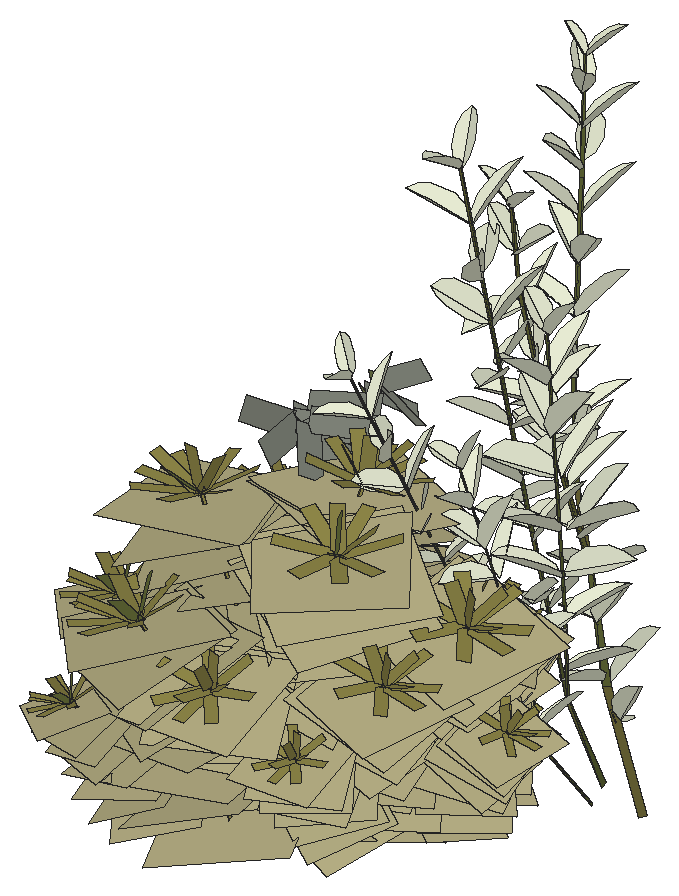
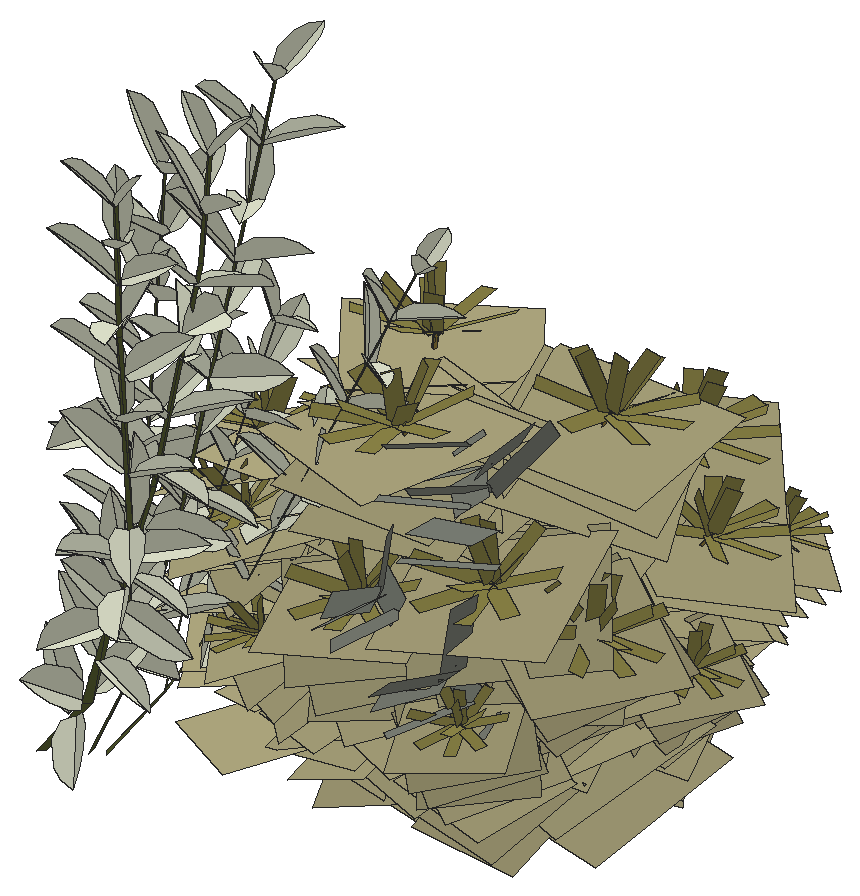
# SketchUp Ruby script. Lengths in inches.
U = 1.inch
M = Sketchup.active_model
def pt(a) = Geom::Point3d.new(a.map { |v| v * U })
def face(e, loops, mat)
  f = e.add_face(loops[0].map { |a| pt(a) })
  loops[1..].each { |l| e.add_face(l.map { |a| pt(a) }).erase! }
  f.material = f.back_material = mat if mat
  f
end
# faces: each face lists its corners as indices into pts; further lists are holes
def faces(e, pts, list, mat = nil) = list.each { |f| face(e, (f[0].is_a?(Array) ? f : [f]).map { |l| l.map { |i| pts[i] } }, mat) }
# xy, xz, yz: faces in a plane at the given z, y or x. An outline is a flat list of corners, or four numbers for a rectangle; further outlines are holes
def ring(l) = l.size == 4 ? [[l[0], l[1]], [l[2], l[1]], [l[2], l[3]], [l[0], l[3]]] : l.each_slice(2).to_a
def flat(e, list, mat, &to3) = list.each { |f| face(e, (f[0].is_a?(Array) ? f : [f]).map { |l| ring(l).map { |u, v| to3.(u, v) } }, mat) }
def xy(e, z, list, mat = nil) = flat(e, list, mat) { |x, y| [x, y, z] }
def xz(e, y, list, mat = nil) = flat(e, list, mat) { |x, z| [x, y, z] }
def yz(e, x, list, mat = nil) = flat(e, list, mat) { |y, z| [x, y, z] }
def lines(e, pts, list) = list.each { |a, b| e.add_line(pt(pts[a]), pt(pts[b])) }
# prism: a flat outline (further loops are holes) pulled along v
def prism(e, loops, v, mat = nil)
  f = face(e, loops, mat); d = Geom::Vector3d.new(v.map { |x| x * U })
  f.pushpull(f.normal.samedirection?(d) ? d.length : -d.length)
end
def box(e, o, s, mat = nil) = prism(e, [[o, [o[0] + s[0], o[1], o[2]], [o[0] + s[0], o[1] + s[1], o[2]], [o[0], o[1] + s[1], o[2]]]], [0, 0, s[2]], mat)
def at(x, y, z, deg = 0) = Geom::Transformation.translation(pt([x, y, z])) * Geom::Transformation.rotation(ORIGIN, Z_AXIS, deg.degrees)
def axes(o, x, y, z) = Geom::Transformation.new([*x, 0, *y, 0, *z, 0, *pt(o).to_a, 1])
def part(name) = M.definitions.add(name)
# library, detail: a bought-in or finely detailed component or shape, given as its bounding box
def library(name, o, s) = part(name).tap { |d| box(d.entities, o, s) }
def detail(e, o, s) = box(e.add_group.entities, o, s)
def put(e, d, t, mat = nil) = e.add_instance(d, t).tap { |i| i.material = mat if mat }
def group(e, t, mat = nil) = e.add_group.tap { |g| g.transformation = t; g.material = mat if mat }.entities
root = M.entities
M.materials.add("Colorsadfasdfa0sd1f06w3").color = [153, 130, 61]
M.materials.add("Euphorbia asdfasd0f150160s159w").color = [180, 173, 131]
M.materials.add("Euphorbiaasdfa0sdf1a56sd016wow Leaf SU").color = [141, 134, 72]
M.materials.add("asdfasdf0165f6asdLeafVar1sfd015as60f1as6").color = [231, 235, 211]
M.materials.add("dw_stemssadfasdfa0sdf1s01d6w1").color = [90, 97, 50]
M.materials.add("viburnumbladsadfasdfad0w122").color = [125, 129, 119]
c1 = part("Component\#315")
p = [[0.25,0,0],[2.05,0.01,0.35],[1.81,4.2,1.66],[0,4.19,1.3125]]
faces(c1.entities,p,[[0,1,2,3]],"viburnumbladsadfasdfad0w122")
c2 = part("viburnumblad2")
put(c2.entities,c1,axes([-19.23,-4.49,-32.18],[83.35428,0,0],[0,79.38502,0],[0,0,83.35428]))
c3 = part("Component\#306")
p = [[4.55,0.11,0],[4.55,0,0],[2.84,0,3.13],[2.84,0.11,3.13],[4.625,0.05,0.04],[2.92,0.05,3.15],
  [2.08,0,8.07],[2.08,0.11,8.07],[2.16,0.05,8.1],[0,0,12.54],[0,0.11,12.54],[0.07,0.05,12.58]]
faces(c3.entities,p,[[0,1,2,3],[1,4,5,2],[1,0,4],[4,0,3,5],[3,2,6,7],[2,5,8,6],[5,3,7,8],[7,6,9,10],
  [6,8,11,9],[8,7,10,11],[10,9,11]],"Colorsadfasdfa0sd1f06w3")
c4 = part("Component\#301")
xy(c4.entities,0,[[0,0,0.7,3.1]],"Euphorbiaasdfa0sdf1a56sd016wow Leaf SU")
c5 = part("Leaf rosette")
put(c5.entities,c4,axes([2.21,1.74,0.13],[-0.4441,0.47879,-0.0956],[-0.4878,-0.4406,0.05935],[-0.03146,0.16757,0.98536]))
put(c5.entities,c4,axes([2.29,1.9,0.17],[-0.62678,-0.10063,-0.18061],[0.01105,-0.59203,0.2915],[-0.31282,0.41486,0.85442]))
put(c5.entities,c4,axes([2.09,1.69,0.1],[-0.10438,0.65169,0],[-0.65169,-0.10438,0],[0,0,1]))
put(c5.entities,c4,axes([1.97,1.77,0.02],[0.31114,0.5228,0.25587],[-0.57125,0.32993,0.02052],[-0.16918,-0.3502,0.92127]))
put(c5.entities,c4,axes([1.93,1.95,0],[0.54816,-0.03215,0.36617],[-0.11878,0.60671,0.23108],[-0.52706,-0.39065,0.75472]))
put(c5.entities,c4,axes([2.04,2.1,0.05],[0.26275,-0.55867,0.23335],[0.34186,0.34684,0.44545],[-0.75711,-0.08556,0.64766]))
put(c5.entities,c4,axes([2.22,2.08,0.13],[-0.29265,-0.59104,-0.02512],[0.40323,-0.2198,0.47401],[-0.65583,0.2952,0.69479]))
c6 = part("Component\#308")
xy(c6.entities,0,[[0,0,5.01,4.64]],"Euphorbia asdfasd0f150160s159w")
c7 = part("Component\#316")
put(c7.entities,c3,at(2.35,3.5,0))
put(c7.entities,c5,at(0.25,1.59,12.45))
put(c7.entities,c6,axes([7.46,0.77,3.64],[0.10848,0.99337,0.03799],[-0.82378,0.11122,-0.55589],[-0.55643,0.02901,0.83038]))
put(c7.entities,c6,axes([1.97,2.58,1.93],[0.80762,-0.50565,0.30344],[0.47433,0.86274,0.17519],[-0.35038,0.00244,0.93661]))
put(c7.entities,c6,axes([5.79,0.14,3.9],[0.5013,0.78918,0.35482],[-0.74775,0.60146,-0.2813],[-0.4354,-0.1243,0.89162]))
put(c7.entities,c6,axes([1.87,2.6,3.75],[0.73154,-0.49698,0.46676],[0.47433,0.86274,0.17519],[-0.48976,0.09324,0.86686]))
put(c7.entities,c6,axes([3.91,7.06,6.66],[-0.50827,-0.83837,-0.19699],[0.8278,-0.53869,0.15675],[-0.23753,-0.08339,0.96779]))
put(c7.entities,c6,axes([1.2,3.99,6.83],[0.56066,-0.79708,0.22433],[0.74237,0.60386,0.29025],[-0.36682,0.0038,0.93028]))
put(c7.entities,c4,axes([2.42,3.73,12.57],[-0.1322,-0.64472,0.04955],[0.10064,0.02944,0.65162],[-0.9678,0.2092,0.14002]))
put(c7.entities,c4,axes([2.57,3.43,12.63],[-0.62833,0.089,-0.18134],[-0.19954,-0.36568,0.51192],[-0.04764,0.82148,0.56824]))
put(c7.entities,c6,axes([4.04,6.92,11.09],[-0.67411,-0.5063,-0.5378],[0.44628,-0.85937,0.24964],[-0.58857,-0.07172,0.80526]))
put(c7.entities,c4,axes([2.5,3.49,12.74],[-0.62833,0.089,-0.18134],[-0.18746,-0.03618,0.63178],[0.11402,0.98935,0.09049]))
put(c7.entities,c4,axes([2.3,3.27,12.51],[0.02916,0.64747,0.12464],[-0.56235,-0.04072,0.34308],[0.5216,-0.18387,0.83314]))
put(c7.entities,c6,axes([0.26,4.96,9.69],[0.33661,-0.92735,0.16343],[0.73504,0.36725,0.56995],[-0.58857,-0.07172,0.80526]))
put(c7.entities,c6,axes([4.76,6.31,12.62],[-0.95056,-0.1129,-0.28929],[0.09021,-0.99179,0.09066],[-0.29715,0.06008,0.95294]))
put(c7.entities,c6,axes([5.2,6.55,10.37],[-0.76372,-0.27738,-0.58291],[0.26517,-0.95808,0.10848],[-0.58857,-0.07172,0.80526]))
c8 = part("Plant stem")
p = [[2.84,0.11,3.13],[2.84,0,3.13],[2.08,0,8.07],[2.08,0.11,8.07],[2.92,0.05,3.15],[2.16,0.05,8.1],
  [0,0,12.54],[0,0.11,12.54],[0.07,0.05,12.58]]
faces(c8.entities,p,[[0,1,2,3],[1,4,5,2],[4,0,3,5],[3,2,6,7],[2,5,8,6],[5,3,7,8],[7,6,8]],"Colorsadfasdfa0sd1f06w3")
c9 = part("Leafy shoot")
put(c9.entities,c8,at(2.35,3.5,0))
put(c9.entities,c5,at(0.25,1.59,12.45))
put(c9.entities,c6,axes([1.87,2.6,3.75],[0.73154,-0.49698,0.46676],[0.47433,0.86274,0.17519],[-0.48976,0.09324,0.86686]))
put(c9.entities,c6,axes([3.91,7.06,6.66],[-0.50827,-0.83837,-0.19699],[0.8278,-0.53869,0.15675],[-0.23753,-0.08339,0.96779]))
put(c9.entities,c6,axes([1.2,3.99,6.83],[0.56066,-0.79708,0.22433],[0.74237,0.60386,0.29025],[-0.36682,0.0038,0.93028]))
put(c9.entities,c4,axes([2.42,3.73,12.57],[-0.1322,-0.64472,0.04955],[0.10064,0.02944,0.65162],[-0.9678,0.2092,0.14002]))
put(c9.entities,c4,axes([2.57,3.43,12.63],[-0.62833,0.089,-0.18134],[-0.19954,-0.36568,0.51192],[-0.04764,0.82148,0.56824]))
put(c9.entities,c6,axes([4.04,6.92,11.09],[-0.67411,-0.5063,-0.5378],[0.44628,-0.85937,0.24964],[-0.58857,-0.07172,0.80526]))
put(c9.entities,c4,axes([2.5,3.49,12.74],[-0.62833,0.089,-0.18134],[-0.18746,-0.03618,0.63178],[0.11402,0.98935,0.09049]))
put(c9.entities,c4,axes([2.3,3.27,12.51],[0.02916,0.64747,0.12464],[-0.56235,-0.04072,0.34308],[0.5216,-0.18387,0.83314]))
put(c9.entities,c6,axes([0.26,4.96,9.69],[0.33661,-0.92735,0.16343],[0.73504,0.36725,0.56995],[-0.58857,-0.07172,0.80526]))
put(c9.entities,c6,axes([4.76,6.31,12.62],[-0.95056,-0.1129,-0.28929],[0.09021,-0.99179,0.09066],[-0.29715,0.06008,0.95294]))
put(c9.entities,c6,axes([5.2,6.55,10.37],[-0.76372,-0.27738,-0.58291],[0.26517,-0.95808,0.10848],[-0.58857,-0.07172,0.80526]))
put(c9.entities,c6,axes([7.03,0.77,3.77],[0.19714,0.84663,0.32426],[-0.94994,0.28899,-0.30484],[-0.2731,-0.45173,0.91532]))
c10 = part("Groundcover plant")
put(c10.entities,c7,axes([0.82,1.83,0.8125],[0.98541,0,-0.17021],[0,1,0],[0.17021,0,0.98541]))
put(c10.entities,c9,axes([4.45,-0.84,-2.24],[0.69527,0.50616,0],[-0.50264,0.69042,-0.10135],[-0.05965,0.08194,0.85401]))
put(c10.entities,c9,axes([1.85,7.37,-3.38],[0.7038,-0.47341,0.14191],[0.46407,0.71797,0.09357],[-0.16999,0,0.84303]))
put(c10.entities,c9,axes([6.9,-3.65,-2.52],[0.79351,0.57769,0],[-0.57366,0.78798,-0.11567],[-0.06808,0.09351,0.97468]))
put(c10.entities,c9,axes([1.36,5.18,-2.66],[0.50674,-0.34086,0.10218],[0.33413,0.51694,0.06737],[-0.12239,0,0.60698]))
put(c10.entities,c9,axes([5.76,-1.49,-2.17],[0.43479,0.43181,0.07251],[-0.43488,0.43544,-0.06951],[-0.06212,-0.06169,0.61918]))
c11 = part("Groundcover clump")
put(c11.entities,c10,axes([25.06,6.72,0.82],[-0.74291,1.22188,0],[-1.22188,-0.74291,0],[0,0,1]))
put(c11.entities,c10,axes([-0.76,2.1875,0.82],[1.43,0,0],[0,1.43,0],[0,0,1]))
put(c11.entities,c10,axes([8.21,24.79,0.82],[-0.6403,-1.27864,0],[1.27864,-0.6403,0],[0,0,1]))
c12 = part("vdw_leaf\#2")
p = [[0,0,0],[-2.77,1.61,2.32],[-4.3125,6.1,4.5],[-3.97,13.49,6.09],[-2.47,18.57,6.3],[-0.2,22.73,5.75],
  [2.54,19.66,6.85],[4.3,15.93,7.09],[5.03,7.6,5.43],[3.32,1.76,2.74]]
faces(c12.entities,p,[[0,1,2,3,4,5],[0,5,6,7,8,9]],"asdfasdf0165f6asdLeafVar1sfd015as60f1as6")
c13 = part("dg_branch_1\#2")
p = [[46.12,1.57,35.62],[46,5.42,35.41],[0.14,1.79,0.05],[0.26,-2.0625,0.27],[74.05,2.99,75.8],[74.11,5.28,75.58],
  [103.46,0.47,94.74],[104.03,2.92,94.84],[81.14,16.92,120.46],[81.2,18.78,120.24],[130.47,-5.6875,130.27],[130.58,-3.66,129.85],
  [80.82,34.4375,191.22],[80.64,35.93,190.9],[148.49,-14.56,203.24],[148.9,-12.8125,203.11],[81.08,37.95,226.93],[81.4,39.1,227.03],
  [157.45,-18.19,250.77],[157.7,-17.01,250.41]]
faces(c13.entities,p,[[0,1,2,3],[4,0,1],[4,1,5],[6,4,5],[6,5,7],[8,4,5],[8,5,9],[10,6,7],
  [10,7,11],[12,8,9],[12,9,13],[14,10,11],[14,11,15],[16,12,13],[16,13,17],[18,14,15],
  [18,15,19]],"dw_stemssadfasdfa0sdf1s01d6w1")
c14 = part("vdw_branch1\#3")
put(c14.entities,c12,axes([120.69,-2.42,117.31],[1.12221,-0.24063,-0.65809],[0.19207,1.24776,-0.12871],[0.65778,0.01392,1.11658]))
put(c14.entities,c12,axes([81,38.9,226.05],[0.7888,-0.58155,0],[0.48308,0.65523,0.47],[-0.28484,-0.38635,0.83138]))
put(c14.entities,c12,axes([78.08,12.69,106.05],[-1.43826,-0.02353,-0.03177],[0.0088,-1.31777,0.57755],[-0.03854,0.57714,1.31741]))
put(c14.entities,c12,axes([130.18,-4.73,130.41],[-0.38031,-1.29044,-0.11242],[1.20662,-0.31032,-0.51987],[0.47109,-0.24694,1.24081]))
put(c14.entities,c12,axes([157.08,-17.89,249.93],[-0.91355,0.40674,0],[-0.37496,-0.84216,0.38752],[0.15762,0.35401,0.92186]))
put(c14.entities,c12,axes([90.64,3.03,86.49],[0.32514,-0.85045,-0.99675],[0.69523,0.98247,-0.61148],[1.11061,-0.36604,0.67459]))
put(c14.entities,c12,axes([80.15,28.42,160.95],[-0.16039,0.95636,-1.06292],[-1.41646,0.03966,0.24943],[0.19509,1.07422,0.93709]))
put(c14.entities,c12,axes([126.74,-5.45,129.22],[-0.59819,0.96152,-0.6841],[-0.85772,0.12575,0.92675],[0.75427,0.88089,0.57856]))
put(c14.entities,c12,axes([133.22,-6.12,150.66],[-0.93823,0.76985,0.59124],[-0.47726,-1.08188,0.65135],[0.84525,0.24366,1.02405]))
put(c14.entities,c12,axes([80.43,22.89,141.32],[-1.42571,-0.19312,0.01373],[0.18338,-1.31425,0.5561],[-0.0621,0.5528,1.32692]))
put(c14.entities,c12,axes([33.14,0.88,26.42],[-0.13338,1.31536,0.04876],[-1.04528,-0.13221,0.7073],[0.72315,0.03348,1.07497]))
put(c14.entities,c12,axes([152.63,-15.08,221.76],[-1.28188,0.41945,0.0579],[-0.3638,-1.18547,0.53367],[0.21665,0.49113,1.23869]))
put(c14.entities,c12,axes([80.05,28.28,160.33],[-0.46732,-1.26661,0.40679],[1.27397,-0.40257,0.21004],[-0.07408,0.44645,1.30501]))
put(c14.entities,c12,axes([153.95,-14.8,235.875],[0.39005,1.07743,0.20605],[-0.96443,0.25296,0.50293],[0.42961,-0.3464,0.99807]))
put(c14.entities,c12,axes([80.2,24.22,141.74],[1.33062,-0.46576,0.02628],[0.44746,1.2746,-0.06608],[-0.00197,0.0722,1.37936]))
put(c14.entities,c12,axes([145.48,-12.5,188.92],[-1.32952,0.16983,0.16138],[-0.09299,-1.2361,0.53471],[0.21503,0.51548,1.22904]))
put(c14.entities,c12,axes([139.64,-9.18,171.24],[0.05682,1.30088,0.23414],[-1.13176,-0.05343,0.57151],[0.58357,-0.22963,1.13417]))
put(c14.entities,c12,axes([70.95,4.35,71.98],[-1.1081,-0.41873,0.64752],[0.33675,-1.28259,-0.25313],[0.6937,-0.04625,1.15721]))
put(c14.entities,c12,axes([59.85,4.55,56.17],[-0.26797,1.24526,0.35754],[-0.9369,-0.41634,0.74783],[0.83377,-0.10389,0.98674]))
put(c14.entities,c12,axes([33.11,3.36,25.66],[-0.57817,-1.07968,-0.5679],[1.11554,-0.21356,-0.7297],[0.49375,-0.78178,0.98363]))
put(c14.entities,c13,at(-0.21,0.34,-0.17),"dw_stemssadfasdfa0sdf1s01d6w1")
put(c14.entities,c12,axes([80.91,19.01,122.53],[-0.84258,1.13222,-0.27981],[-1.15093,-0.75138,0.42537],[0.18861,0.47293,1.3457]))
put(c14.entities,c12,axes([119.8,-1.22,114.1],[-1.3235,-0.25012,0.09101],[0.25933,-1.31572,0.15537],[0.05991,0.1698,1.33794]))
put(c14.entities,c12,axes([46.29,5.1,38.04],[0.98937,0.73827,-0.47585],[-0.72359,1.03721,0.10473],[0.44068,0.18581,1.20453]))
put(c14.entities,c12,axes([81.1875,33.03,184.45],[1.33883,0.26986,0.35053],[-0.09581,1.22087,-0.57399],[-0.42216,0.53228,1.20262]))
put(c14.entities,c12,axes([80.16,36.28,206.98],[-0.83993,0.85737,-0.6234],[-1.05964,-0.65701,0.5241],[0.02941,0.81391,1.07976]))
put(c14.entities,c12,axes([154.86,-16.15,234.87],[0.02509,-1.15302,-0.28506],[1.1487,-0.04894,0.29908],[-0.30202,-0.28195,1.11384]))
put(c14.entities,c12,axes([108.77,-0.33,101.14],[-0.47691,-1.03266,-0.72709],[1.25395,-0.29455,-0.40416],[0.15052,-0.81814,1.06325]))
put(c14.entities,c12,axes([89.79,3.01,85.87],[-0.61344,0.75518,0.8965],[-0.17758,-1.01824,0.73622],[1.13385,0.22574,0.58569]))
put(c14.entities,c12,axes([81.56,20.31,123.29],[0.37259,-1.3435,0.21057],[1.29385,0.32364,-0.22445],[0.16906,0.25791,1.34638]))
put(c14.entities,c12,axes([46.45,1.82,36.74],[-0.77883,0.29892,1.0614],[0.19124,-1.24314,0.49044],[1.08598,0.43329,0.67484]))
put(c14.entities,c12,axes([71.37,4.02,72.32],[0.72905,0.81546,-0.74421],[-0.66805,0.98958,0.42988],[0.8391,0.14186,0.97745]))
put(c14.entities,c12,axes([136.59,-5.88,150.53],[0.85845,-0.99897,-0.12437],[0.96526,0.81273,0.13453],[-0.02572,-0.18182,1.28292]))
put(c14.entities,c12,axes([80.375,38.8,225.86],[-0.25178,0.96778,0],[-0.89216,-0.23211,0.38752],[0.37503,0.09757,0.92186]))
put(c14.entities,c12,axes([74.43,7.99,85.38],[-1.05703,0.91669,-0.33543],[-0.95806,-0.87958,0.61531],[0.18697,0.6754,1.25659]))
put(c14.entities,c12,axes([76.57,9.74,89.32],[0.63146,-1.21538,0.33508],[1.18148,0.49387,-0.43517],[0.26321,0.48577,1.26593]))
put(c14.entities,c12,axes([81.6875,36.97,207.4],[0.09422,-1.04424,0.38486],[1.01646,0.1939,0.27727],[-0.33299,0.33382,0.98727]))
put(c14.entities,c12,axes([157.29,-17.17,249.98],[0.50586,-0.50586,0],[0.38853,0.38853,0.41105],[-0.29684,-0.29684,0.56115]))
put(c14.entities,c12,axes([79.92,15.8,106.09],[1.03917,-0.29343,-0.90675],[-0.14587,1.22131,-0.5624],[0.92163,0.5191,0.88824]))
put(c14.entities,c12,axes([61.95,3.88,56.26],[0.41243,-1.28546,0],[1.17466,0.37688,-0.54831],[0.5221,0.16751,1.23363]))
put(c14.entities,c12,axes([151.99,-14.79,208.15],[-0.48571,-1.21723,-0.32393],[1.25386,-0.50033,0],[-0.12005,-0.30087,1.31056]))
put(c14.entities,c12,axes([108.44,0.62,102.22],[0.82183,0.96078,0.38967],[-0.62327,0.08618,1.10203],[0.79141,-0.88661,0.51693]))
put(c14.entities,c12,axes([145.6,-10.56,188.62],[1.03241,-0.02554,-0.82693],[0.3944,1.11584,0.45794],[0.70325,-0.61672,0.89706]))
put(c14.entities,c12,axes([78.59,32.3,183.89],[-1.12675,-0.42036,0.43987],[0.5899,-0.98149,0.57312],[0.14901,0.70693,1.05726]))
put(c14.entities,c12,axes([152.08,-13.42,223.37],[0.79993,-0.44251,-0.69938],[0.68456,0.82615,0.26026],[0.41048,-0.60953,0.85515]))
put(c14.entities,c12,axes([140.71,-8.74,170.55],[0.41903,-1.24177,-0.32393],[1.26224,0.33728,0.33986],[-0.23168,-0.40836,1.26573]))
put(c14.entities,c12,axes([149.25,-12.53,205.78],[1.24456,0.38285,0.23414],[-0.42999,1.04826,0.57151],[-0.02056,-0.62679,1.13417]))
c15 = part("vdw_leaf\#3")
p = [[0,0,0],[-2.77,1.61,2.32],[-4.3125,6.1,4.5],[-3.97,13.49,6.09],[-2.47,18.57,6.3],[-0.2,22.73,5.75],
  [2.54,19.66,6.85],[4.3,15.93,7.09],[5.03,7.6,5.43],[3.32,1.76,2.74]]
faces(c15.entities,p,[[0,1,2,3,4,5],[0,5,6,7,8,9]],"asdfasdf0165f6asdLeafVar1sfd015as60f1as6")
c16 = part("dw_brancj_2\#2")
p = [[9.7,-0.22,29.95],[0.23,-1.96,0.34],[-0.05,1.51,0.11],[9.65,1.51,29.46],[18.64,-8.75,84.43],[18.96,-6.63,84.625],
  [1.53,6.02,63.68],[1.42,8.18,63.25],[-10.58,8.77,161.17],[-10.41,9.98,160.68],[26.34,-9.37,211.72],[26.57,-8.28,211.23]]
faces(c16.entities,p,[[0,1,2],[0,2,3],[4,0,3],[4,3,5],[6,0,3],[6,3,7],[8,6,7],[8,7,9],
  [10,4,5],[10,5,11]],"dw_stemssadfasdfa0sdf1s01d6w1")
c17 = part("vdw_branch2\#3")
put(c17.entities,c15,axes([19.53,-5.9,102.42],[1.12377,-0.50004,0],[0.46097,1.03596,0.47664],[-0.19377,-0.43548,1.13389]))
put(c17.entities,c15,axes([-5.89,6.52,109.44],[-1.07209,0.83679,0],[-0.77141,-0.98832,0.52702],[0.32427,0.41545,1.25373]))
put(c17.entities,c15,axes([-0.44,8.23,75.28],[0.88709,-0.9947,0],[0.92159,0.82189,0.33087],[-0.25219,-0.22491,1.26111]))
put(c17.entities,c15,axes([24.71,-8.97,190.81],[-0.82641,0.91101,0],[-0.83983,-0.76184,0.47664],[0.35303,0.32025,1.13389]))
put(c17.entities,c15,axes([-2.29,8.24,91.35],[1.24603,-0.47303,0],[0.43826,1.15445,0.33087],[-0.11993,-0.31592,1.26111]))
put(c17.entities,c15,axes([12.26,-3.11,37.92],[-0.64625,1.02205,0.22511],[-1.04383,-0.61044,-0.22511],[-0.07533,-0.30931,1.18809]))
put(c17.entities,c15,axes([26.17,-9.17,210.27],[-0.99452,-0.10453,0],[0.09636,-0.91681,0.38752],[-0.04051,0.38539,0.92186]))
put(c17.entities,c15,axes([-6.07,9.4,125.35],[-0.90214,-0.98107,0],[0.90896,-0.83583,0.33087],[-0.24874,0.22873,1.26111]))
put(c17.entities,c15,axes([-4.13,7.29,110.58],[0.44715,-1.078,0.64369],[1.05816,0.63649,0.33087],[-0.58725,0.40856,1.09216]))
put(c17.entities,c15,axes([23.91,-8.22,171.96],[0.62307,0.85009,-0.63406],[-0.71531,0.8798,0.47664],[0.78296,0.12729,0.94004]))
put(c17.entities,c16,at(-0.09,0.18,-0.25),"dw_stemssadfasdfa0sdf1s01d6w1")
put(c17.entities,c15,axes([23.34,-9.65,156.59],[-0.31364,-1.00782,0.58216],[1.10369,-0.17062,0.29925],[-0.17137,0.6239,0.98776]))
put(c17.entities,c15,axes([15.03,-3.37,58.83],[-1.05425,-0.00194,0.58442],[-0.14303,-1.11707,-0.26172],[0.55355,-0.3046,0.99755]))
put(c17.entities,c15,axes([-11.625,9.46,160.37],[0.36812,0.92978,0],[-0.85713,0.33936,0.38752],[0.3603,-0.14265,0.92186]))
put(c17.entities,c15,axes([21.32,-8.53,138.72],[1.21379,0.19904,0],[-0.19904,1.21379,0],[0,0,1.23]))
put(c17.entities,c15,axes([22.54,-9.2,141.43],[-1.02887,0.17955,0.60182],[-0.23387,-1.13057,-0.06253],[0.56696,-0.17376,1.02111]))
put(c17.entities,c15,axes([23.9,-8.82,173.84],[-1.14567,-0.37474,0],[0.35918,-1.0981,0.04438],[-0.01409,0.04308,1.17993]))
put(c17.entities,c15,axes([-7.84,8.92,143.59],[-1.26971,0.40522,0],[-0.37543,-1.17638,0.33087],[0.10274,0.32192,1.26111]))
put(c17.entities,c15,axes([19.77,-8.01,85.98],[-0.32405,-1.14591,0.18674],[1.10278,-0.32969,-0.10948],[0.15845,0.14442,1.16117]))
put(c17.entities,c15,axes([-0.62,5.76,76.34],[-0.08879,1.17576,-0.67771],[-1.34525,-0.16582,-0.11144],[-0.17897,0.66309,1.17383]))
put(c17.entities,c15,axes([20.49,-8.22,121.07],[0.39924,-0.78471,-0.8233],[1.08735,0.33121,0.2116],[0.09035,-0.83005,0.83495]))
put(c17.entities,c15,axes([15.15,-3.72,62.9],[1.16251,0.40128,-0.0211],[-0.39924,1.16074,0.07874],[0.0456,-0.06757,1.2273]))
put(c17.entities,c15,axes([20.72,-8.08,120.26],[-0.03693,1.2277,-0.06551],[-1.22944,-0.03698,0],[-0.00197,0.06548,1.22825]))
put(c17.entities,c15,axes([22.58,-8.36,155.57],[-0.56247,1.09386,0],[-1.00839,-0.51852,0.47664],[0.42389,0.21796,1.13389]))
put(c17.entities,c15,axes([3.97,3.13,57.96],[-1.09459,0.76041,0],[-0.72262,-1.0402,-0.1735],[-0.10109,-0.14552,1.29352]))
put(c17.entities,c15,axes([-10.8,9.06,160.75],[-0.66334,-0.72138,0],[0.66835,-0.61458,0.24329],[-0.1829,0.16818,0.92729]))
put(c17.entities,c15,axes([19.06,-9.3125,103.96],[-1.01345,0.25553,-0.60051],[-0.2265,-1.12952,-0.09839],[-0.59598,0.03076,1.01889]))
put(c17.entities,c15,axes([18.07,-6.2,81.7],[-0.56247,1.09386,0],[-1.00839,-0.51852,0.47664],[0.42389,0.21796,1.13389]))
put(c17.entities,c15,axes([12.95,-0.39,43.31],[0.13044,-1.19832,0],[1.11025,0.12085,0.29925],[-0.30382,-0.03307,1.14057]))
put(c17.entities,c15,axes([2.28,8.28,56.18],[1.32413,-0.31027,0],[0.30923,1.31968,-0.11144],[0.02542,0.1085,1.35543]))
put(c17.entities,c15,axes([-7.55,9.96,143.07],[1.34251,-0.21744,0],[0.20045,1.23761,0.52702],[-0.08426,-0.52024,1.25373]))
put(c17.entities,c15,axes([26.15,-8.25,210.66],[0.94661,-0.25364,0],[0.235,0.87703,0.24329],[-0.06431,-0.24,0.92729]))
put(c17.entities,c15,axes([-6.48,11.37,125.16],[0.64635,1.10315,0.46356],[-1.16569,0.46153,0.52702],[0.27017,-0.6478,1.16488]))
put(c17.entities,c15,axes([25.74,-8.35,191.28],[0.13044,-1.19832,0],[1.11025,0.12085,0.29925],[-0.30382,-0.03307,1.14057]))
put(c17.entities,c15,axes([-5.125,7.47,91.6],[-1.10024,0.63688,0.48318],[-0.78682,-1.00808,-0.46292],[0.14137,-0.65404,1.184]))
put(root,c2,axes([2221.18,267.54,27.9],[-0.00309,0.00736,0.0079],[-0.00654,-0.00921,0.0057],[0.00929,-0.00262,0.00521]))
put(root,c2,axes([2218.01,271.63,26.87],[0.00481,-0.00941,-0.00652],[0.01076,0.00809,-0.00374],[0.00656,-0.00389,0.01045]))
put(root,c2,axes([2221.03,270.42,19.84],[-0.00141,0.01241,-0.00136],[-0.00618,0.00049,0.01093],[0.01085,0.0019,0.00605]))
put(root,c2,axes([2218.66,271.95,17.35],[0.00148,-0.01296,0.00142],[0.00776,-0.00002,-0.00823],[0.00903,0.00196,0.00851]))
put(root,c2,axes([2218.91,278.3,26.51],[0.00523,-0.00868,-0.00226],[0.00529,0.00516,-0.00737],[0.00696,0.00241,0.00605]))
put(root,c2,axes([2219.75,278.16,27.57],[0.00677,-0.00276,-0.00724],[0.0003,0.00981,-0.00339],[0.00756,0.00183,0.00557]))
put(root,c2,axes([2219.78,277.77,25.67],[-0.00435,-0.00477,0.00798],[0.00611,-0.00825,-0.00162],[0.00685,0.00405,0.00535]))
put(root,c2,axes([2219.26,271.94,19.07],[0.00627,-0.00896,-0.00619],[0.00573,0.0092,-0.00751],[0.00942,0.00088,0.00827]))
put(root,c2,axes([2220.97,277.38,26.42],[-0.00677,0.00276,0.00724],[0.00154,-0.00908,0.00464],[0.00741,0.00415,0.00458]))
put(root,c2,axes([2220.34,271.72,20.4375],[0.00745,-0.00026,-0.01011],[-0.00018,0.01255,-0.00046],[0.01011,0.00042,0.00745]))
put(root,c2,axes([2220.11,272.03,17.86],[-0.00427,-0.00859,0.00811],[0.00683,-0.00794,-0.00482],[0.00917,0.00302,0.00803]))
put(root,c2,axes([2219.59,271.62,27.68],[-0.00288,-0.01252,-0.00147],[0.01138,-0.00177,-0.00721],[0.00645,-0.00276,0.01087]))
put(root,c2,axes([2221.22,270.84,28.35],[-0.00909,-0.00791,0.00471],[0.00591,-0.01009,-0.00553],[0.00706,-0.00173,0.0107]))
put(root,c2,axes([2220.41,278.5625,26.53],[0.00062,-0.00952,0.00405],[0.00764,-0.00238,-0.00656],[0.00666,0.00333,0.00596]))
put(root,c2,axes([2221.69,271.29,18.7],[-0.00745,0.00026,0.01011],[0.00262,-0.01208,0.00224],[0.00977,0.00344,0.00711]))
put(root,c2,axes([2222.57,267.54,28.43],[-0.00733,-0.00034,0.00907],[-0.00172,-0.01154,-0.00184],[0.00876,-0.00225,0.00608]))
put(root,c2,axes([2220.05,271.28,29.4],[0.00501,-0.0098,-0.00679],[0.00996,0.00749,-0.00346],[0.00656,-0.00389,0.01045]))
put(root,c2,axes([2220.76,268.77,29.29],[0.0022,-0.00655,-0.00816],[0.00813,0.00764,-0.00386],[0.00785,-0.0054,0.00541]))
put(root,c2,axes([2221.01,272.59,19.29],[0.00141,-0.01241,0.00136],[0.00862,-0.00002,-0.00914],[0.00903,0.00196,0.00851]))
put(root,c2,axes([2222.29,268.67,29.38],[-0.00278,-0.01118,-0.00257],[0.00839,-0.00011,-0.00838],[0.00753,-0.00365,0.00688]))
put(root,c2,axes([2223.71,267.68,29.41],[-0.00715,-0.00814,0.0046],[0.00423,-0.00805,-0.00746],[0.00803,-0.00268,0.00677]))
put(root,c2,axes([2222.86,267.88,30.59],[0.00322,-0.00766,-0.00823],[0.00813,0.00764,-0.00386],[0.00755,-0.0046,0.00633]))
put(root,c11,axes([2211.35,243.65,7.84],[1.49047,0,0],[0,1.49047,0],[0,0,1.49047]))
put(root,c14,axes([2245.37,272.43,7.1875],[-0.11174,0.0797,0],[-0.0797,-0.11174,0],[0,0,0.16889]))
put(root,c17,axes([2242.33,271.16,7.57],[-0.10096,-0.0593,-0.07152],[0.0662,-0.11272,0],[-0.05012,-0.02944,0.14408]))
put(root,c17,axes([2242.19,272.51,8.3],[-0.15667,-0.0351,-0.03733],[0.03572,-0.15945,0],[-0.0296,-0.00663,0.19757]))
